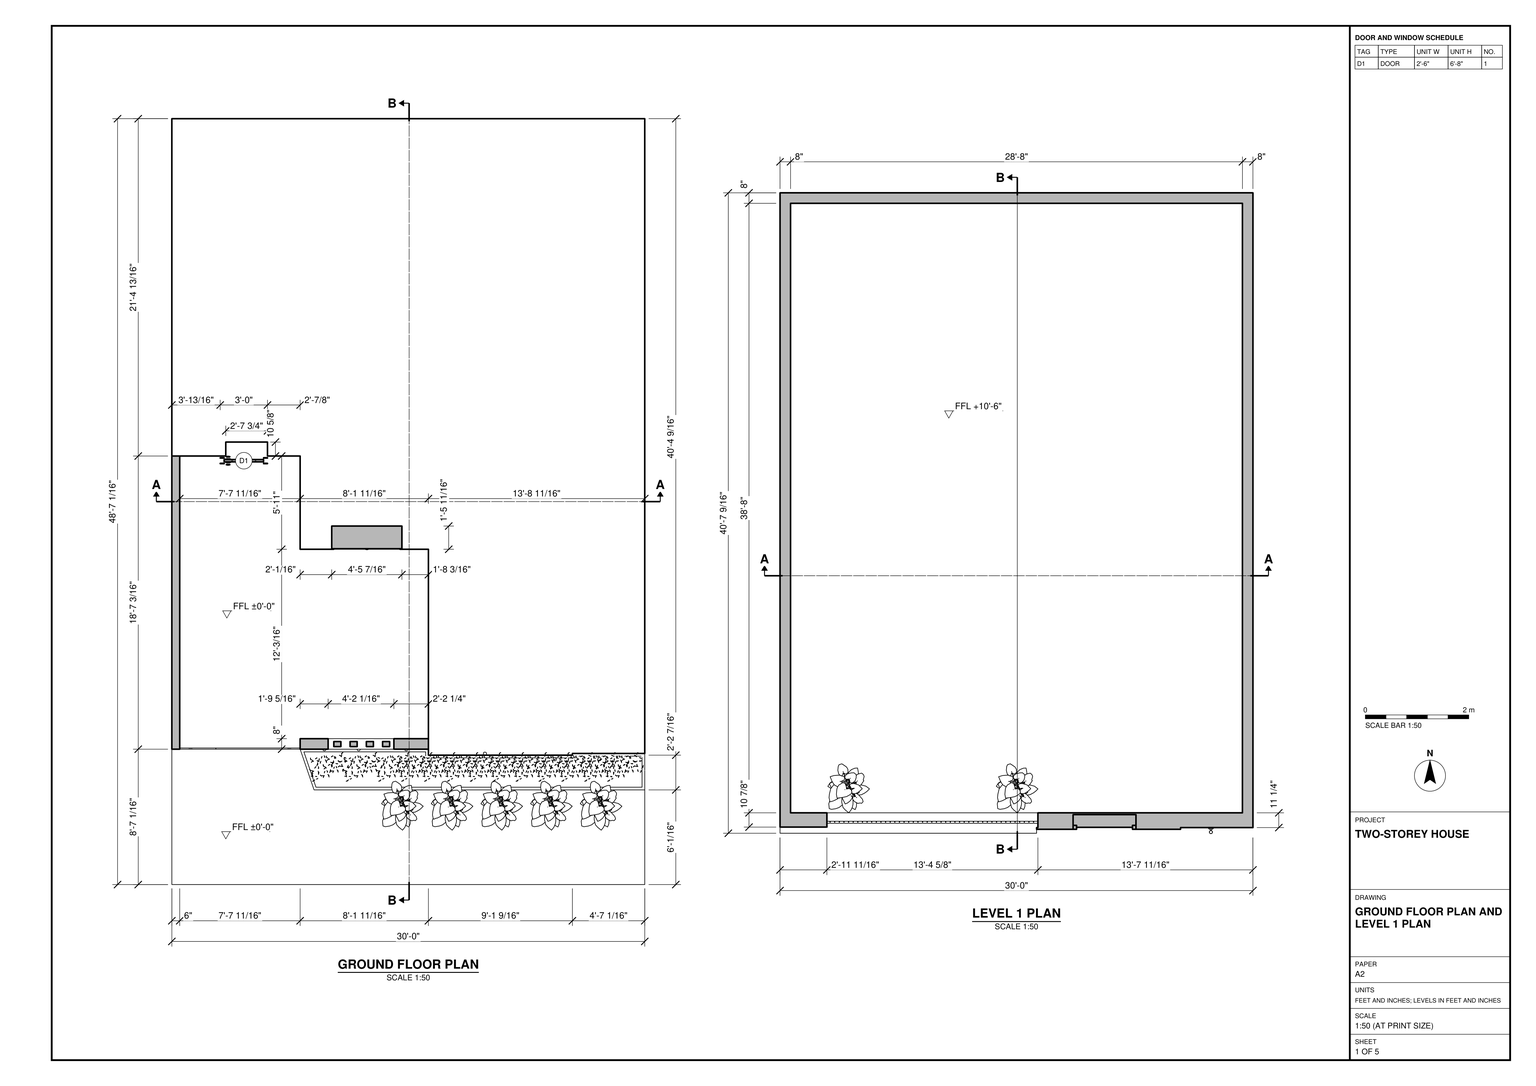
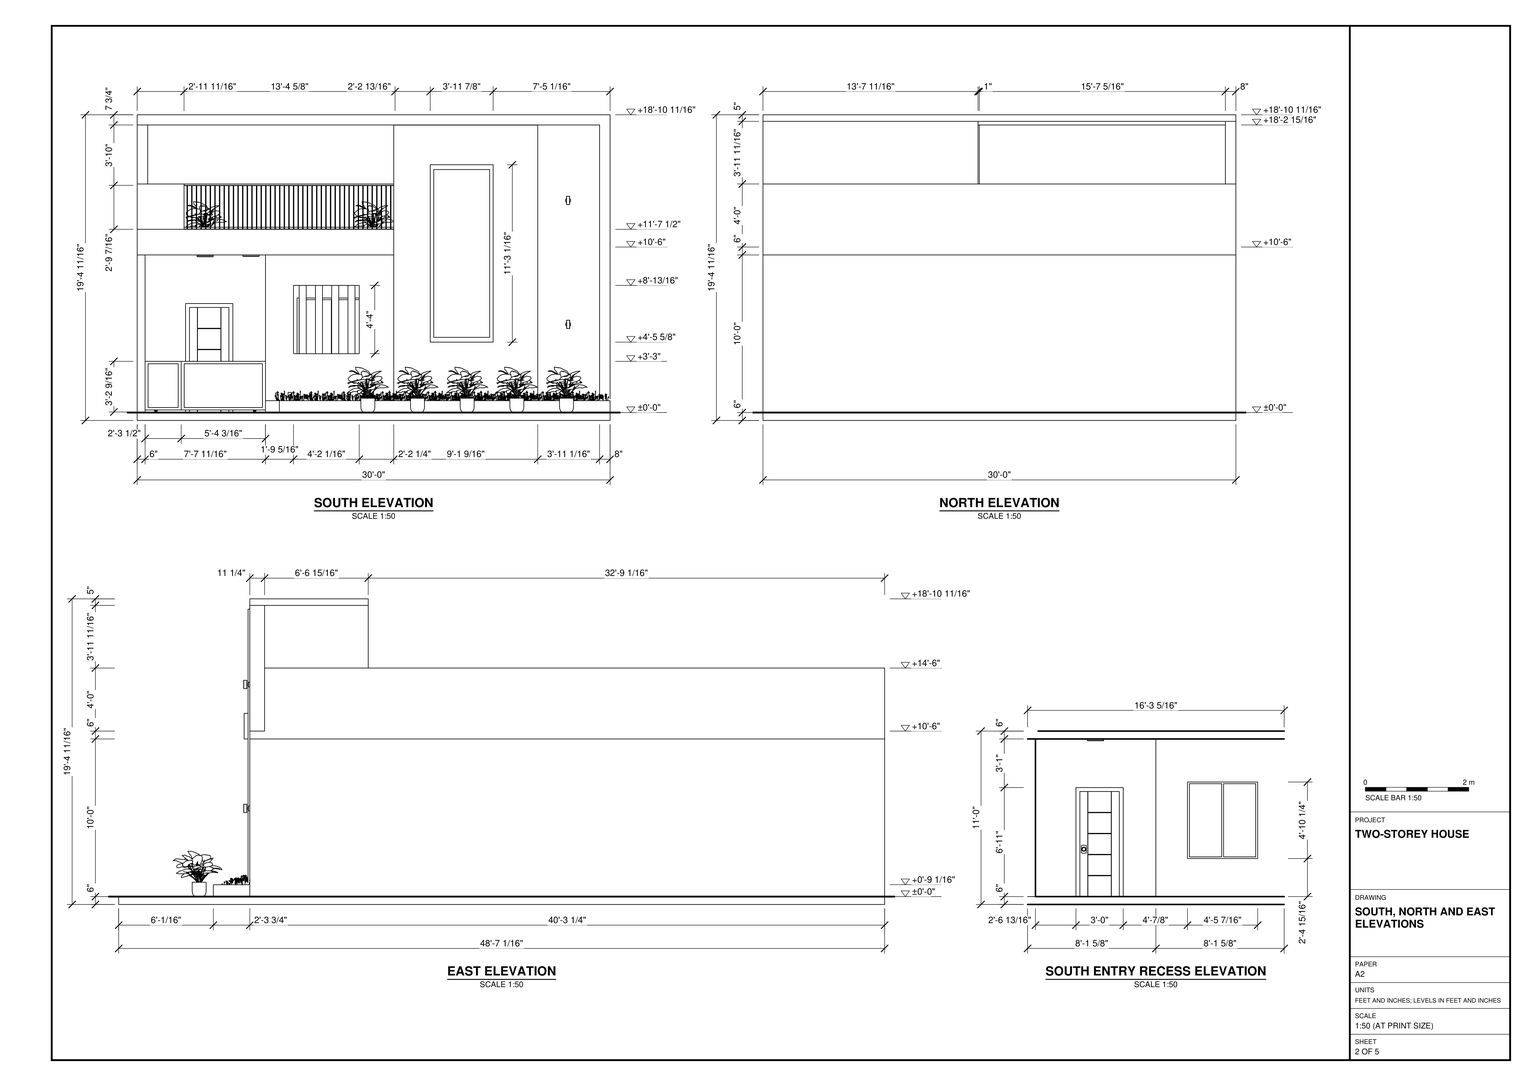
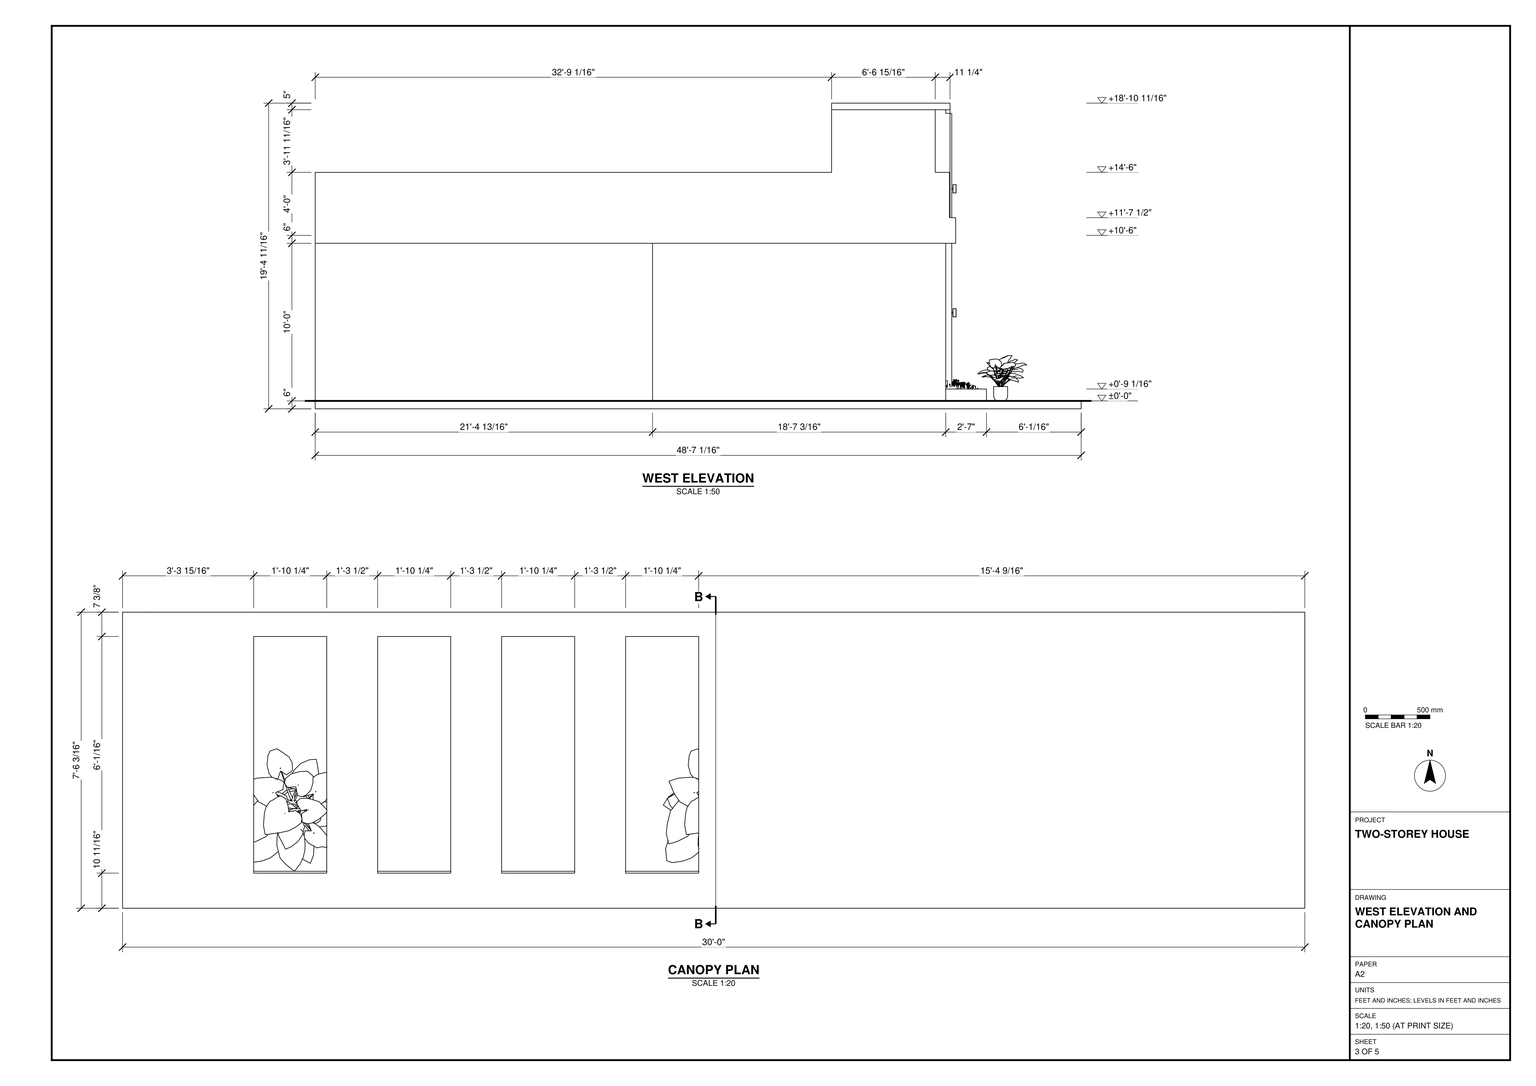
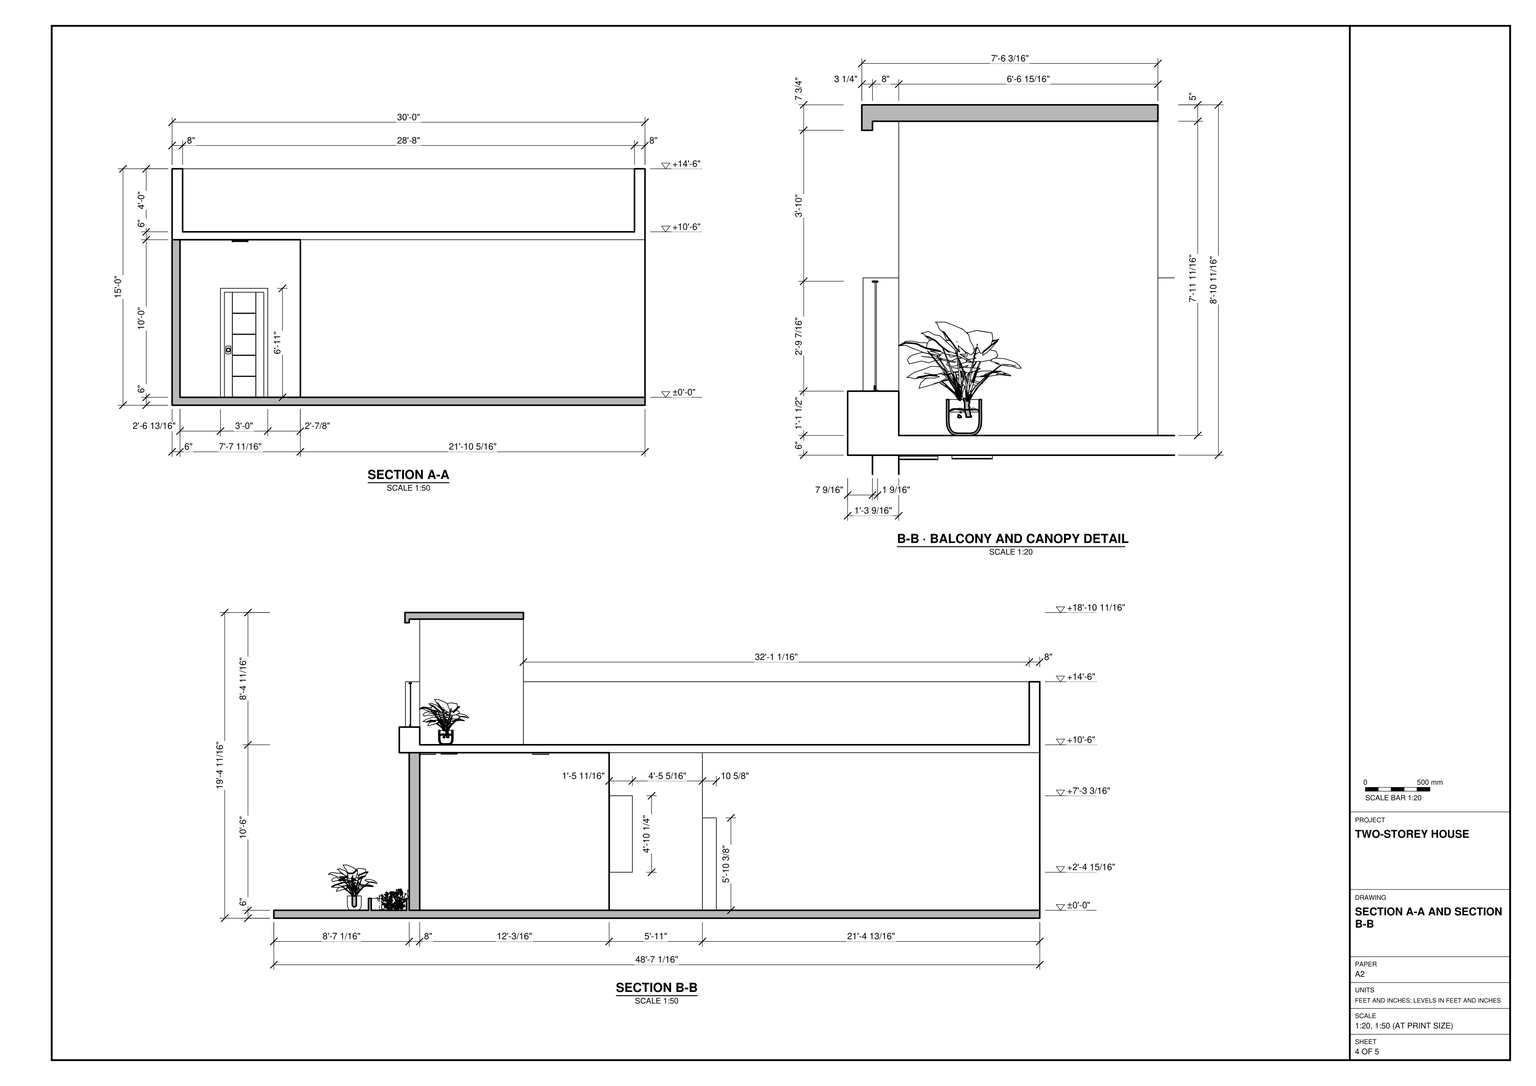
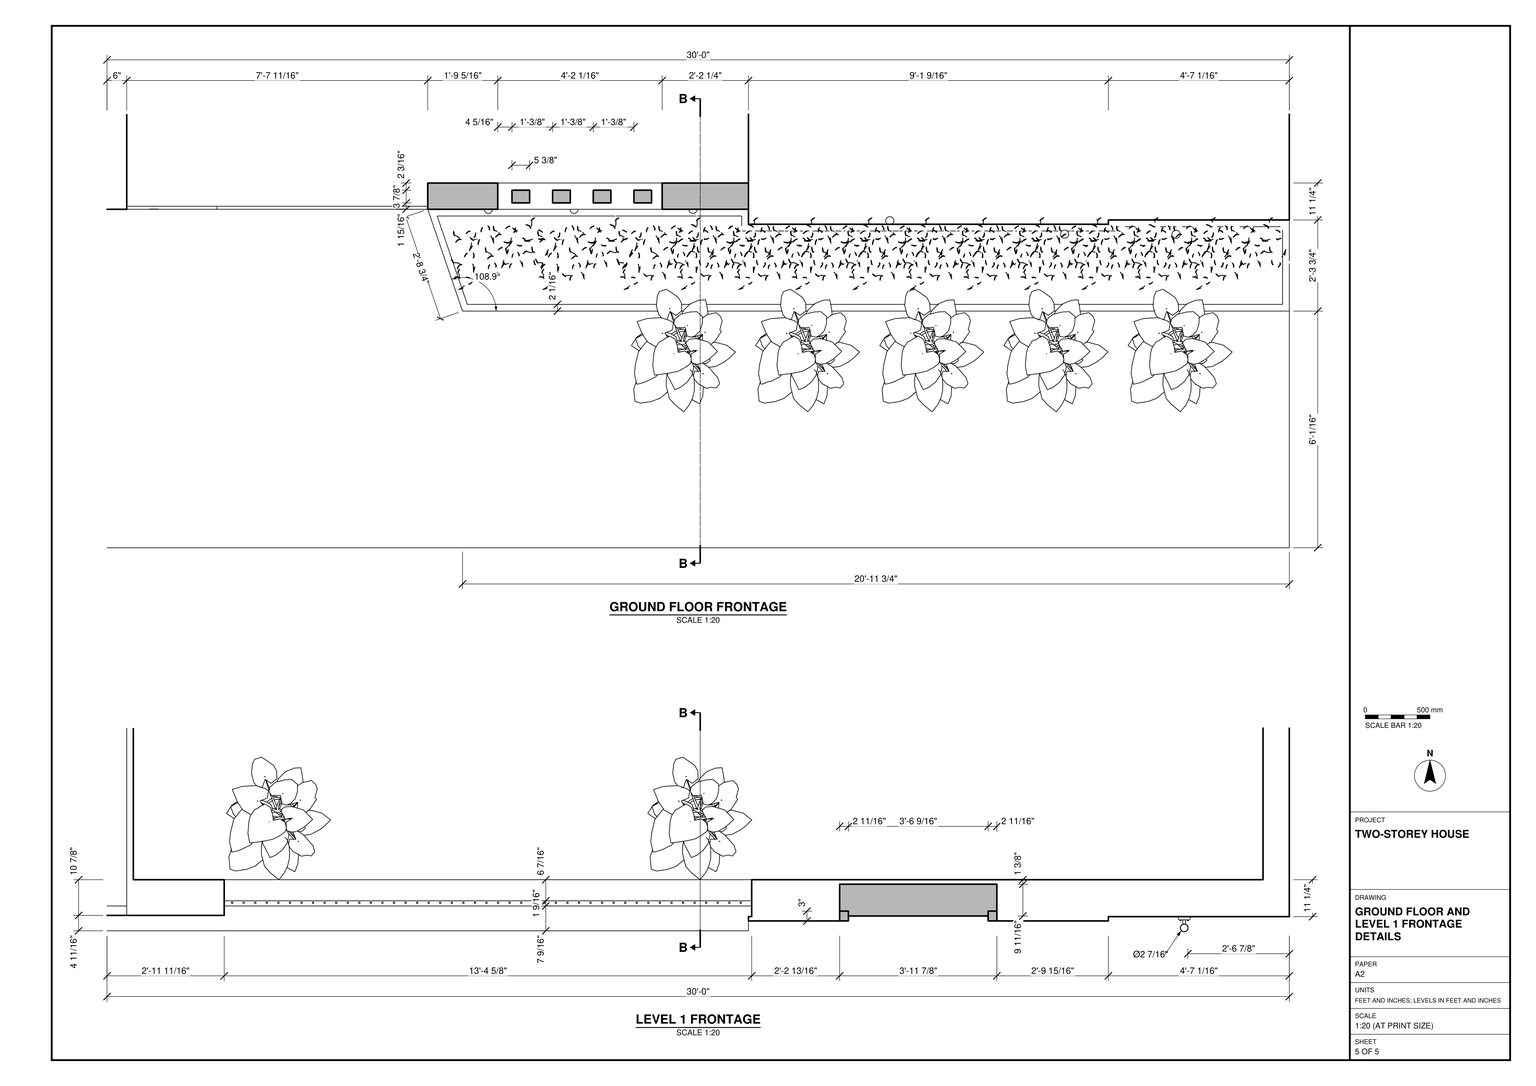
Build the house shown in task_files/diagram_01.pdf in SketchUp. Work in feet and inches. Including the front approach and projecting elements, the overall model must measure 30'-1 1/4" wide by 48'-7 1/16" deep by 19'-4 11/16" high. Set the ground floor at ±0'-0" and the upper terrace floor at +10'-6".

Use the ground floor plan to lay out the base slab, the stepped walls of the south entry recess and the approach from the gate. Follow the wall and slab thicknesses shown. Set the entrance door back beneath the terrace, with the divided window to its right. Distinguish these recessed elements from the gate, the vertical screen and the tall framed panel seen in the south elevation.

Build the upper slab with its perimeter parapets. Use the side elevations to locate the change in wall height near the south end. Run the canopy across the front, with four rectangular openings over the railed part of the terrace and a solid portion to the right. Place the planting strip and pots along the frontage and include the terrace plants and lights where shown. Plants, lights and other loose or decorative items may be any suitable library components.

Keep walls, slabs, parapets, the canopy and each joinery or furniture piece in separate groups or components. Use components for repeated parts. Save one SketchUp model as output_files/two_storey_house_with_a_slotted_terrace_canopy.skp.

# SketchUp Ruby script. Lengths in inches.
U = 1.inch
M = Sketchup.active_model
def pt(a) = Geom::Point3d.new(a.map { |v| v * U })
def face(e, loops, mat)
  f = e.add_face(loops[0].map { |a| pt(a) })
  loops[1..].each { |l| e.add_face(l.map { |a| pt(a) }).erase! }
  f.material = f.back_material = mat if mat
  f
end
# faces: each face lists its corners as indices into pts; further lists are holes
def faces(e, pts, list, mat = nil) = list.each { |f| face(e, (f[0].is_a?(Array) ? f : [f]).map { |l| l.map { |i| pts[i] } }, mat) }
# xy, xz, yz: faces in a plane at the given z, y or x. An outline is a flat list of corners, or four numbers for a rectangle; further outlines are holes
def ring(l) = l.size == 4 ? [[l[0], l[1]], [l[2], l[1]], [l[2], l[3]], [l[0], l[3]]] : l.each_slice(2).to_a
def flat(e, list, mat, &to3) = list.each { |f| face(e, (f[0].is_a?(Array) ? f : [f]).map { |l| ring(l).map { |u, v| to3.(u, v) } }, mat) }
def xy(e, z, list, mat = nil) = flat(e, list, mat) { |x, y| [x, y, z] }
def xz(e, y, list, mat = nil) = flat(e, list, mat) { |x, z| [x, y, z] }
def yz(e, x, list, mat = nil) = flat(e, list, mat) { |y, z| [x, y, z] }
def lines(e, pts, list) = list.each { |a, b| e.add_line(pt(pts[a]), pt(pts[b])) }
# prism: a flat outline (further loops are holes) pulled along v
def prism(e, loops, v, mat = nil)
  f = face(e, loops, mat); d = Geom::Vector3d.new(v.map { |x| x * U })
  f.pushpull(f.normal.samedirection?(d) ? d.length : -d.length)
end
def box(e, o, s, mat = nil) = prism(e, [[o, [o[0] + s[0], o[1], o[2]], [o[0] + s[0], o[1] + s[1], o[2]], [o[0], o[1] + s[1], o[2]]]], [0, 0, s[2]], mat)
def at(x, y, z, deg = 0) = Geom::Transformation.translation(pt([x, y, z])) * Geom::Transformation.rotation(ORIGIN, Z_AXIS, deg.degrees)
def axes(o, x, y, z) = Geom::Transformation.new([*x, 0, *y, 0, *z, 0, *pt(o).to_a, 1])
def part(name) = M.definitions.add(name)
# library, detail: a bought-in or finely detailed component or shape, given as its bounding box
def library(name, o, s) = part(name).tap { |d| box(d.entities, o, s) }
def detail(e, o, s) = box(e.add_group.entities, o, s)
def put(e, d, t, mat = nil) = e.add_instance(d, t).tap { |i| i.material = mat if mat }
def group(e, t, mat = nil) = e.add_group.tap { |g| g.transformation = t; g.material = mat if mat }.entities
root = M.entities
M.materials.add("2").color = [128, 128, 128]
M.materials["2"].alpha = 0.5
M.materials.add("Aluminum_Anodized_Clear").color = [178, 178, 174]
M.materials.add("[0047_Khaki]").color = [240, 230, 140]
M.materials.add("[0050_LemonChiffon]").color = [255, 250, 205]
M.materials.add("[0118_Thistle]").color = [216, 191, 216]
M.materials.add("[0134_DimGray]").color = [105, 105, 105]
M.materials.add("[0137_Black]").color = [0, 0, 0]
M.materials.add("[Color_007]").color = [58, 58, 58]
M.materials.add("[Field Rectangle Tile]").color = [196, 189, 179]
M.materials.add("[Slate]").color = [102, 110, 108]
M.materials.add("[Translucent_Glass_Green_Dark]").color = [69, 69, 69]
M.materials["[Translucent_Glass_Green_Dark]"].alpha = 0.9
c1 = part("b01\#3")
box(c1.entities,[0,9.84,0.59],[1.57,143.7,0.2],"Aluminum_Anodized_Clear")
c2 = part("b01\#2")
prism(c2.entities,[[[0.98,153.54,0.59],[0,153.54,0.59],[0,153.54,0.79],[0.79,153.54,0.79],[0.79,153.54,2.17],[0.98,153.54,2.17]]],[0,-143.7,0],"Aluminum_Anodized_Clear")
c3 = part("Square bar")
box(c3.entities,[0,0,0],[0.39,0.39,33.07])
c4 = part("01")
g1 = group(c4.entities,at(-246.49,-73.84,116.14))
put(g1,c1,at(0,0,32.68))
put(g1,c2,at(0,0,-0.59))
put(g1,c3,at(0.39,55.91,0.2),"Aluminum_Anodized_Clear")
put(g1,c3,at(0.39,115.75,0.2),"Aluminum_Anodized_Clear")
put(g1,c3,at(0.39,68.5,0.2),"Aluminum_Anodized_Clear")
put(g1,c3,at(0.39,96.85,0.2),"Aluminum_Anodized_Clear")
put(g1,c3,at(0.39,65.35,0.2),"Aluminum_Anodized_Clear")
put(g1,c3,at(0.39,43.31,0.2),"Aluminum_Anodized_Clear")
put(g1,c3,at(0.39,71.65,0.2),"Aluminum_Anodized_Clear")
put(g1,c3,at(0.39,112.6,0.2),"Aluminum_Anodized_Clear")
put(g1,c3,at(0.39,128.35,0.2),"Aluminum_Anodized_Clear")
put(g1,c3,at(0.39,144.09,0.2),"Aluminum_Anodized_Clear")
put(g1,c3,at(0.39,27.56,0.2),"Aluminum_Anodized_Clear")
put(g1,c3,at(0.39,137.8,0.2),"Aluminum_Anodized_Clear")
put(g1,c3,at(0.39,21.26,0.2),"Aluminum_Anodized_Clear")
put(g1,c3,at(0.39,109.45,0.2),"Aluminum_Anodized_Clear")
put(g1,c3,at(0.39,62.2,0.2),"Aluminum_Anodized_Clear")
put(g1,c3,at(0.39,100,0.2),"Aluminum_Anodized_Clear")
put(g1,c3,at(0.39,14.96,0.2),"Aluminum_Anodized_Clear")
put(g1,c3,at(0.39,106.3,0.2),"Aluminum_Anodized_Clear")
put(g1,c3,at(0.39,90.55,0.2),"Aluminum_Anodized_Clear")
put(g1,c3,at(0.39,87.4,0.2),"Aluminum_Anodized_Clear")
put(g1,c3,at(0.39,74.8,0.2),"Aluminum_Anodized_Clear")
put(g1,c3,at(0.39,131.5,0.2),"Aluminum_Anodized_Clear")
put(g1,c3,at(0.39,40.16,0.2),"Aluminum_Anodized_Clear")
put(g1,c3,at(0.39,52.76,0.2),"Aluminum_Anodized_Clear")
put(g1,c3,at(0.39,118.9,0.2),"Aluminum_Anodized_Clear")
put(g1,c3,at(0.39,33.86,0.2),"Aluminum_Anodized_Clear")
put(g1,c3,at(0.39,24.41,0.2),"Aluminum_Anodized_Clear")
put(g1,c3,at(0.39,46.46,0.2),"Aluminum_Anodized_Clear")
put(g1,c3,at(0.39,11.8125,0.2),"Aluminum_Anodized_Clear")
put(g1,c3,at(0.39,77.95,0.2),"Aluminum_Anodized_Clear")
put(g1,c3,at(0.39,49.61,0.2),"Aluminum_Anodized_Clear")
put(g1,c3,at(0.39,125.2,0.2),"Aluminum_Anodized_Clear")
put(g1,c3,at(0.39,84.25,0.2),"Aluminum_Anodized_Clear")
put(g1,c3,at(0.39,103.15,0.2),"Aluminum_Anodized_Clear")
put(g1,c3,at(0.39,81.1,0.2),"Aluminum_Anodized_Clear")
put(g1,c3,at(0.39,93.7,0.2),"Aluminum_Anodized_Clear")
put(g1,c3,at(0.39,134.65,0.2),"Aluminum_Anodized_Clear")
put(g1,c3,at(0.39,150.39,0.2),"Aluminum_Anodized_Clear")
put(g1,c3,at(0.39,30.71,0.2),"Aluminum_Anodized_Clear")
put(g1,c3,at(0.39,59.06,0.2),"Aluminum_Anodized_Clear")
put(g1,c3,at(0.39,122.05,0.2),"Aluminum_Anodized_Clear")
put(g1,c3,at(0.39,147.24,0.2),"Aluminum_Anodized_Clear")
put(g1,c3,at(0.39,37.01,0.2),"Aluminum_Anodized_Clear")
put(g1,c3,at(0.39,140.94,0.2),"Aluminum_Anodized_Clear")
put(g1,c3,at(0.39,18.11,0.2),"Aluminum_Anodized_Clear")
c5 = part("Untitled")
xy(c5.entities,0,[[207.4375,0,243.4375,3]],"[Color_007]")
xy(c5.entities,2,[[209.4375,0,241.4375,1.5],[209.4375,1.5,241.4375,3]],"[Color_007]")
xy(c5.entities,71.9375,[[209.4375,0,241.4375,1.5],[209.4375,1.5,241.4375,3]],"[Color_007]")
xy(c5.entities,73.9375,[[207.4375,0,243.4375,3]],"[Color_007]")
xz(c5.entities,0,[[[207.4375,0,243.4375,73.9375],[209.4375,2,241.4375,71.9375]]],"[Color_007]")
xz(c5.entities,1.5,[[209.4375,2,241.4375,71.9375]],"[Translucent_Glass_Green_Dark]")
xz(c5.entities,3,[[[207.4375,0,243.4375,73.9375],[209.4375,2,241.4375,71.9375]]],"[Color_007]")
yz(c5.entities,207.4375,[[0,0,3,73.9375]],"[Color_007]")
yz(c5.entities,209.4375,[[0,2,1.5,71.9375],[1.5,2,3,71.9375]],"[Color_007]")
yz(c5.entities,241.4375,[[0,2,1.5,71.9375],[1.5,2,3,71.9375]],"[Color_007]")
yz(c5.entities,243.4375,[[0,0,3,73.9375]],"[Color_007]")
c6 = part("WindowDoubleBlack")
xy(c6.entities,0,[[0,0,96.0625,1.57]],"[0137_Black]")
xy(c6.entities,2.71,[[2.71,0,46.85,1.57],[49.41,0,93.35,1.57]],"[0137_Black]")
xy(c6.entities,122.09,[[2.71,0,46.85,1.57],[49.41,0,50,1.57],[50,0,93.35,1.57]],"[0137_Black]")
xy(c6.entities,124.8,[[0,0,96.0625,1.57]],"[0137_Black]")
xz(c6.entities,0,[[[0,0,96.0625,124.8],[2.71,2.71,46.85,122.09],[49.41,2.71,93.35,122.09]]],"[0137_Black]")
xz(c6.entities,1.57,[[2.71,2.71,46.85,122.09],[49.41,2.71,93.35,122.09]],"2")
xz(c6.entities,1.57,[[[0,0,96.0625,124.8],[2.71,2.71,46.85,122.09],[49.41,2.71,93.35,122.09]]],"[0137_Black]")
yz(c6.entities,0,[[0,0,1.57,124.8]],"[0137_Black]")
yz(c6.entities,2.71,[[0,2.71,1.57,122.09]],"[0137_Black]")
yz(c6.entities,46.85,[[0,2.71,1.57,122.09]],"[0137_Black]")
yz(c6.entities,49.41,[[0,2.71,1.57,122.09]],"[0137_Black]")
yz(c6.entities,93.35,[[0,2.71,1.57,122.09]],"[0137_Black]")
yz(c6.entities,96.0625,[[0,0,1.57,124.8]],"[0137_Black]")
c7 = library("Untitled (14)",[0,0,0],[7.13,36,83])
c8 = library("GATE DESIGN",[0,0,0],[157.48,1.97,82.05])
c9 = library("Lamp Wall Outdoor 94-02",[-1.89,-4.65,-3.17],[3.78,4.65,6.35])
c10 = library("Heliconia_psittacorum",[-112.89,55.56,-1.2],[171.96,175.92,51.58])
c11 = library("Lamp Ceiling 114-44",[-1.26,-1.26,-3.9375],[2.52,2.52,3.9375])
c12 = library("Dome Light",[-12,-12,0],[24,24,12])
c13 = library("Indoor Plant 001",[-24.46,-30.5625,0],[48.74,57.4,53.14])
c14 = library("Tlon Light 950 Ceiling 152 008",[-18.7,-18.7,-3.78],[37.4,37.4,3.56])
xy(root,-6,[[0,0,360,583.0625]])
xy(root,0,[[109.71,74.11,357.96,74.11,357.96,97.77,306.95,97.77,306.95,96.46,193.27,96.46,193.27,101.02,100.52,101.02],[195.3125,98.5,195.3125,255.25,97.66,255.25,97.66,326.25,72.81,326.25,72.81,336.875,41.06,336.875,41.06,326.25,0,326.25,0,583.0625,360,583.0625,360,99.8125,304.91,99.8125,304.91,98.5],[97.66,103.0625,195.3125,111.0625]])
xy(root,0,[[0,0,360,0,360,72.0625,108.25,72.0625,97.66,103.0625,97.66,111.0625,195.3125,111.0625,195.3125,255.25,97.66,255.25,97.66,326.25,72.81,326.25,72.81,336.875,41.06,336.875,41.06,326.25,6,326.25,6,103.0625,0,103.0625]],"[Slate]")
xy(root,9.0625,[[[108.25,72.0625,360,72.0625,360,99.8125,304.91,99.8125,304.91,98.5,195.3125,98.5,195.3125,103.0625,97.66,103.0625],[109.71,74.11,100.52,101.02,193.27,101.02,193.27,96.46,306.95,96.46,306.95,97.77,357.96,97.77,357.96,74.11]]])
xy(root,28.96,[[121.7,255.25,175.14,272.9375]])
xy(root,44.81,[[[118.97,103.0625,169.03,111.0625],[123.31,105.01,128.68,108.88],[135.68,105.01,141.06,108.88],[148.06,105.01,153.43,108.88],[160.43,105.01,165.81,108.88]]],"[0134_DimGray]")
xy(root,53.6,[[223.08,98.5,270.96,109.6875]],"[0118_Thistle]")
xy(root,70.375,[[41.06,326.25,72.81,336.875]])
xy(root,87.21,[[121.7,255.25,175.14,272.9375]])
xy(root,96.81,[[118.97,103.0625,169.03,111.0625]])
xy(root,97.87,[[148.06,105.01,153.43,108.88]])
xy(root,99.24,[[160.43,105.01,165.81,108.88]])
xy(root,99.31,[[123.31,105.01,128.68,108.88]])
xy(root,100.93,[[135.68,105.01,141.06,108.88]])
xy(root,120,[[0,95.5,0,103.0625,6,103.0625,6,98.5,97.66,98.5,97.66,103.0625,195.3125,103.0625,195.3125,95.5],[6,98.5,6,326.25,97.66,326.25,97.66,255.25,195.3125,255.25,195.3125,111.0625,97.66,111.0625,97.66,98.5],[0,103.0625,6,326.25],[97.66,103.0625,195.3125,111.0625]])
xy(root,126,[[8,111.0625,352,575.0625]])
xy(root,139.5,[[0,95.5,195.3125,95.5,195.3125,99.8125,196.3,99.8125,196.3,111.0625,35.67,111.0625,35.67,100.1875,0,100.1875]],"[0047_Khaki]")
xy(root,174,[[352,111.0625,360,111.0625,360,583.0625,0,583.0625,0,189.97,8,189.97,8,575.0625,352,575.0625]])
xy(root,174,[[0,100.1875,35.67,111.0625]],"[0047_Khaki]")
xy(root,188.66,[[223.08,98.5,270.96,109.6875]])
xy(root,218.8125,[[195.3125,98.5,304.91,99.8125]])
xy(root,218.9375,[[0,99.8125,196.3,103.0625]])
xy(root,221.6875,[[[0,103.0625,0,111.0625,8,111.0625,8,189.97,360,189.97,360,111.0625,196.3,111.0625,196.3,103.0625],[39.92,110.51,62.17,182.57],[77.67,110.51,99.92,182.57],[115.42,110.51,137.67,182.57],[153.17,110.51,175.42,182.57]],[0,111.0625,8,189.97]])
xy(root,226.6875,[[[0,99.8125,360,189.97],[39.92,110.51,62.17,182.57],[77.67,110.51,99.92,182.57],[115.42,110.51,137.67,182.57],[153.17,110.51,175.42,182.57]]])
xz(root,0,[[0,-6,360,0]])
xz(root,72.0625,[[108.25,0,360,9.0625]])
xz(root,74.11,[[109.71,0,357.96,9.0625]])
xz(root,95.5,[[0,120,195.3125,139.5]],"[0047_Khaki]")
xz(root,96.46,[[193.27,0,306.95,9.0625]])
xz(root,97.77,[[306.95,0,352,9.0625],[352,0,357.96,9.0625]])
xz(root,98.5,[[195.3125,0,304.91,9.0625]])
xz(root,98.5,[[[195.3125,9.0625,304.91,218.8125],[223.08,53.6,270.96,188.66]]],"[0118_Thistle]")
xz(root,99.8125,[[304.91,0,352,9.0625],[352,0,360,9.0625],[352,9.0625,360,9.0625,360,226.6875,0,226.6875,0,218.9375,352,218.9375],[195.3125,139.5,196.3,218.8125]])
xz(root,99.8125,[[304.91,9.0625,352,9.0625,352,218.9375,196.3,218.9375,196.3,218.8125,304.91,218.8125]],"[Field Rectangle Tile]")
xz(root,100.1875,[[0,139.5,35.67,174]],"[0047_Khaki]")
xz(root,101.02,[[100.52,0,193.27,9.0625]])
xz(root,103.0625,[[0,0,6,120],[97.66,0,195.3125,9.0625],[0,218.9375,196.3,221.6875]])
xz(root,103.0625,[[[97.66,9.0625,195.3125,120],[118.97,44.81,169.03,96.81]]],"[Field Rectangle Tile]")
xz(root,105.01,[[123.31,44.81,128.68,99.31],[135.68,44.81,141.06,100.93],[148.06,44.81,153.43,97.87],[160.43,44.81,165.81,99.24]],"[0134_DimGray]")
xz(root,108.88,[[123.31,44.81,128.68,99.31],[135.68,44.81,141.06,100.93],[148.06,44.81,153.43,97.87],[160.43,44.81,165.81,99.24]],"[0134_DimGray]")
xz(root,109.6875,[[223.08,53.6,270.96,188.66]],"[0118_Thistle]")
xz(root,110.51,[[39.92,221.6875,62.17,226.6875],[77.67,221.6875,99.92,226.6875],[115.42,221.6875,137.67,226.6875],[153.17,221.6875,175.42,226.6875]])
xz(root,111.0625,[[[97.66,0,195.3125,120],[118.97,44.81,169.03,96.81]],[8,126,8,174,35.67,174,35.67,139.5,196.3,139.5,196.3,126],[196.3,126,196.3,221.6875,360,221.6875,360,174,352,174,352,126]])
xz(root,111.0625,[[0,174,8,221.6875]],"[0118_Thistle]")
xz(root,182.57,[[39.92,221.6875,62.17,226.6875],[77.67,221.6875,99.92,226.6875],[115.42,221.6875,137.67,226.6875],[153.17,221.6875,175.42,226.6875]])
xz(root,189.97,[[0,221.6875,360,226.6875]])
xz(root,189.97,[[0,174,8,221.6875]],"[0118_Thistle]")
xz(root,255.25,[[[97.66,0,195.3125,120],[121.7,28.96,175.14,87.21]]],"[0050_LemonChiffon]")
xz(root,272.9375,[[121.7,28.96,175.14,87.21]],"[0050_LemonChiffon]")
xz(root,326.25,[[0,0,6,120]])
xz(root,326.25,[[6,0,41.06,0,41.06,70.375,72.81,70.375,72.81,0,97.66,0,97.66,120,6,120]],"[0050_LemonChiffon]")
xz(root,336.875,[[41.06,0,72.81,70.375]])
xz(root,575.0625,[[8,126,352,174]])
xz(root,583.0625,[[0,-6,360,0],[0,0,360,120],[0,120,360,174]])
yz(root,0,[[0,-6,0,0,103.0625,0,103.0625,120,326.25,120,326.25,0,583.0625,0,583.0625,-6],[326.25,0,583.0625,120],[99.8125,218.9375,103.0625,221.6875],[99.8125,221.6875,189.97,226.6875]])
yz(root,0,[[95.5,120,95.5,139.5,100.1875,139.5,100.1875,174,111.0625,174,111.0625,221.6875,189.97,221.6875,189.97,174,583.0625,174,583.0625,120]],"[0118_Thistle]")
yz(root,6,[[103.0625,0,326.25,120]],"[0050_LemonChiffon]")
yz(root,8,[[189.97,126,575.0625,174]])
yz(root,8,[[111.0625,126,189.97,221.6875]],"[0118_Thistle]")
yz(root,35.67,[[100.1875,139.5,111.0625,174]])
yz(root,39.92,[[110.51,221.6875,182.57,226.6875]])
yz(root,41.06,[[326.25,0,336.875,70.375]])
yz(root,62.17,[[110.51,221.6875,182.57,226.6875]])
yz(root,72.81,[[326.25,0,336.875,70.375]])
yz(root,77.67,[[110.51,221.6875,182.57,226.6875]])
yz(root,97.66,[[255.25,0,326.25,120]],"[0050_LemonChiffon]")
yz(root,97.66,[[103.0625,0,111.0625,120]],"[0134_DimGray]")
yz(root,99.92,[[110.51,221.6875,182.57,226.6875]])
yz(root,115.42,[[110.51,221.6875,182.57,226.6875]])
yz(root,118.97,[[103.0625,44.81,111.0625,96.81]],"[0134_DimGray]")
yz(root,121.7,[[255.25,28.96,272.9375,87.21]])
yz(root,123.31,[[105.01,44.81,108.88,99.31]],"[0134_DimGray]")
yz(root,128.68,[[105.01,44.81,108.88,99.31]],"[0134_DimGray]")
yz(root,135.68,[[105.01,44.81,108.88,100.93]],"[0134_DimGray]")
yz(root,137.67,[[110.51,221.6875,182.57,226.6875]])
yz(root,141.06,[[105.01,44.81,108.88,100.93]],"[0134_DimGray]")
yz(root,148.06,[[105.01,44.81,108.88,97.87]],"[0134_DimGray]")
yz(root,153.17,[[110.51,221.6875,182.57,226.6875]])
yz(root,153.43,[[105.01,44.81,108.88,97.87]],"[0134_DimGray]")
yz(root,160.43,[[105.01,44.81,108.88,99.24]],"[0134_DimGray]")
yz(root,165.81,[[105.01,44.81,108.88,99.24]],"[0134_DimGray]")
yz(root,169.03,[[103.0625,44.81,111.0625,96.81]],"[0134_DimGray]")
yz(root,175.14,[[255.25,28.96,272.9375,87.21]],"[0050_LemonChiffon]")
yz(root,175.42,[[110.51,221.6875,182.57,226.6875]])
yz(root,193.27,[[96.46,0,101.02,9.0625]])
yz(root,195.3125,[[98.5,0,103.0625,9.0625],[103.0625,0,111.0625,120],[95.5,120,98.5,139.5]])
yz(root,195.3125,[[98.5,139.5,99.8125,218.8125]],"[0047_Khaki]")
yz(root,195.3125,[[111.0625,0,255.25,120]],"[0050_LemonChiffon]")
yz(root,195.3125,[[98.5,9.0625,103.0625,120]],"[0118_Thistle]")
yz(root,196.3,[[99.8125,139.5,99.8125,218.9375,103.0625,218.9375,103.0625,221.6875,111.0625,221.6875,111.0625,139.5]],"[0047_Khaki]")
yz(root,223.08,[[98.5,53.6,109.6875,188.66]],"[0118_Thistle]")
yz(root,270.96,[[98.5,53.6,109.6875,188.66]],"[0118_Thistle]")
yz(root,304.91,[[98.5,0,99.8125,9.0625],[98.5,9.0625,99.8125,218.8125]])
yz(root,306.95,[[96.46,0,97.77,9.0625]])
yz(root,352,[[111.0625,126,575.0625,174]])
yz(root,357.96,[[74.11,0,97.77,9.0625]])
yz(root,360,[[0,-6,583.0625,-6,583.0625,0,99.8125,0,99.8125,9.0625,72.0625,9.0625,72.0625,0,0,0],[99.8125,0,583.0625,120],[99.8125,120,583.0625,120,583.0625,174,111.0625,174,111.0625,126,99.8125,126],[99.8125,126,111.0625,221.6875],[99.8125,221.6875,189.97,226.6875]])
p = [[97.66,103.0625,0],[108.25,72.0625,0],[108.25,72.0625,9.0625],[97.66,103.0625,9.0625],[109.71,74.11,0],[100.52,101.02,0],
  [100.52,101.02,9.0625],[109.71,74.11,9.0625]]
faces(root,p,[[0,1,2,3],[4,5,6,7]])
put(root,c4,axes([107.2,-141.85,23.36],[0,-1,0],[1.11775,0,0],[0,0,1]))
put(root,c5,axes([-52.78,98.5,53.6],[1.32986,0,0],[0,1,0],[0,0,1.82671]))
put(root,c6,axes([121.7,255.25,28.96],[0.55628,0,0],[0,0.26,0],[0,0,0.46674]))
put(root,c7,at(72.81,319.12,0,90))
put(root,c8,axes([6,103.0625,0.44],[0.58202,0,0],[0,0.47,0],[0,0,0.47]))
put(root,c9,at(328.09,99.8125,67.14))
put(root,c9,at(328,99.8125,161.49))
put(root,c10,axes([165.87,99.23,0.38],[0,0.32,0],[-0.32,0,0],[0,0,0.32]))
put(root,c10,axes([191.49,99.23,0.38],[0,0.32,0],[-0.32,0,0],[0,0,0.32]))
put(root,c10,axes([216.24,99.23,0.38],[0,0.32,0],[-0.32,0,0],[0,0,0.32]))
put(root,c10,axes([233.67,99.23,0.38],[0,0.32,0],[-0.32,0,0],[0,0,0.32]))
put(root,c10,axes([251.09,99.23,0.38],[0,0.32,0],[-0.32,0,0],[0,0,0.32]))
put(root,c10,axes([268.52,99.23,0.38],[0,0.32,0],[-0.32,0,0],[0,0,0.32]))
put(root,c10,axes([285.94,99.23,0.38],[0,0.32,0],[-0.32,0,0],[0,0,0.32]))
put(root,c10,axes([303.37,99.23,0.38],[0,0.32,0],[-0.32,0,0],[0,0,0.32]))
put(root,c10,axes([320.79,99.23,0.38],[0,0.32,0],[-0.32,0,0],[0,0,0.32]))
put(root,c10,axes([338.22,99.23,0.38],[0,0.32,0],[-0.32,0,0],[0,0,0.32]))
put(root,c10,axes([355.64,99.23,0.38],[0,0.32,0],[-0.32,0,0],[0,0,0.32]))
put(root,c10,axes([373.07,99.23,0.38],[0,0.32,0],[-0.32,0,0],[0,0,0.32]))
put(root,c10,axes([390.49,99.23,0.38],[0,0.32,0],[-0.32,0,0],[0,0,0.32]))
put(root,c11,at(116.12,103.0625,15.37))
put(root,c11,at(142.22,103.0625,14.27))
put(root,c11,at(178.41,103.0625,14.31))
put(root,c11,at(238.35,99.59,12.39))
put(root,c11,at(291.57,95.47,13.12))
put(root,c11,at(325.52,95.47,13.12))
put(root,c12,at(-23.62,250.38,0))
put(root,c13,axes([175.57,61.26,0],[0.65,0,0],[0,0.65,0],[0,0,0.65]))
put(root,c13,axes([213.38,61.26,0],[0.65,0,0],[0,0.65,0],[0,0,0.65]))
put(root,c13,axes([251.2,61.26,0],[0.65,0,0],[0,0.65,0],[0,0,0.65]))
put(root,c13,axes([289.01,61.26,0],[0.65,0,0],[0,0.65,0],[0,0,0.65]))
put(root,c13,axes([326.82,61.26,0],[0.65,0,0],[0,0.65,0],[0,0,0.65]))
put(root,c13,axes([52.29,130.93,126],[0.65,0,0],[0,0.65,0],[0,0,0.65]))
put(root,c13,axes([180.55,130.93,126],[0.65,0,0],[0,0.65,0],[0,0,0.65]))
put(root,c14,axes([51.71,289.53,119.85],[0.33,0,0],[0,0.33,0],[0,0,0.33]))
put(root,c14,axes([51.71,203.18,119.85],[0.33,0,0],[0,0.33,0],[0,0,0.33]))
put(root,c14,axes([51.71,116.84,119.85],[0.33,0,0],[0,0.33,0],[0,0,0.33]))
put(root,c14,axes([86.63,133.42,120.07],[0.33,0,0],[0,0.33,0],[0,0,0.33]))
